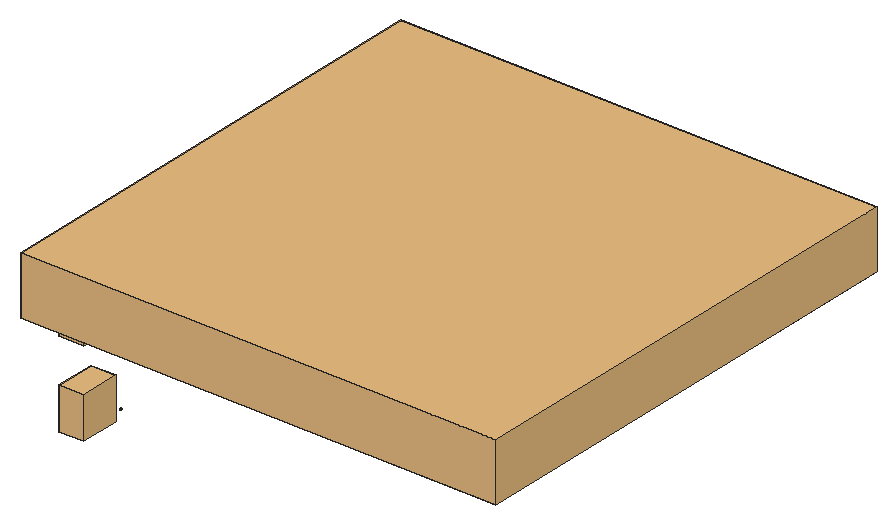
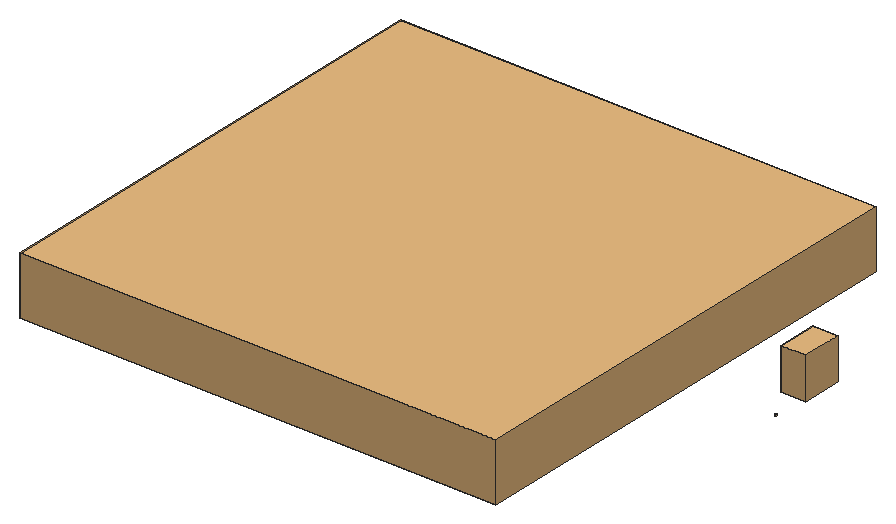
# SketchUp Ruby script. Lengths in inches.
U = 1.inch
M = Sketchup.active_model
def pt(a) = Geom::Point3d.new(a.map { |v| v * U })
def face(e, loops, mat)
  f = e.add_face(loops[0].map { |a| pt(a) })
  loops[1..].each { |l| e.add_face(l.map { |a| pt(a) }).erase! }
  f.material = f.back_material = mat if mat
  f
end
# faces: each face lists its corners as indices into pts; further lists are holes
def faces(e, pts, list, mat = nil) = list.each { |f| face(e, (f[0].is_a?(Array) ? f : [f]).map { |l| l.map { |i| pts[i] } }, mat) }
# xy, xz, yz: faces in a plane at the given z, y or x. An outline is a flat list of corners, or four numbers for a rectangle; further outlines are holes
def ring(l) = l.size == 4 ? [[l[0], l[1]], [l[2], l[1]], [l[2], l[3]], [l[0], l[3]]] : l.each_slice(2).to_a
def flat(e, list, mat, &to3) = list.each { |f| face(e, (f[0].is_a?(Array) ? f : [f]).map { |l| ring(l).map { |u, v| to3.(u, v) } }, mat) }
def xy(e, z, list, mat = nil) = flat(e, list, mat) { |x, y| [x, y, z] }
def xz(e, y, list, mat = nil) = flat(e, list, mat) { |x, z| [x, y, z] }
def yz(e, x, list, mat = nil) = flat(e, list, mat) { |y, z| [x, y, z] }
def lines(e, pts, list) = list.each { |a, b| e.add_line(pt(pts[a]), pt(pts[b])) }
# prism: a flat outline (further loops are holes) pulled along v
def prism(e, loops, v, mat = nil)
  f = face(e, loops, mat); d = Geom::Vector3d.new(v.map { |x| x * U })
  f.pushpull(f.normal.samedirection?(d) ? d.length : -d.length)
end
def box(e, o, s, mat = nil) = prism(e, [[o, [o[0] + s[0], o[1], o[2]], [o[0] + s[0], o[1] + s[1], o[2]], [o[0], o[1] + s[1], o[2]]]], [0, 0, s[2]], mat)
def at(x, y, z, deg = 0) = Geom::Transformation.translation(pt([x, y, z])) * Geom::Transformation.rotation(ORIGIN, Z_AXIS, deg.degrees)
def axes(o, x, y, z) = Geom::Transformation.new([*x, 0, *y, 0, *z, 0, *pt(o).to_a, 1])
def part(name) = M.definitions.add(name)
# library, detail: a bought-in or finely detailed component or shape, given as its bounding box
def library(name, o, s) = part(name).tap { |d| box(d.entities, o, s) }
def detail(e, o, s) = box(e.add_group.entities, o, s)
def put(e, d, t, mat = nil) = e.add_instance(d, t).tap { |i| i.material = mat if mat }
def group(e, t, mat = nil) = e.add_group.tap { |g| g.transformation = t; g.material = mat if mat }.entities
root = M.entities
M.materials.add("green").color = [174, 139, 102]
M.materials.add("vio").color = [206, 114, 100]
c1 = library("3DGeom~121_Defintion",[-425.32,-500,-417.04],[850.64,1000,834.08])
c2 = part("3DGeom~122_Defintion")
p = [[-352.95,-477.04,-406.33],[-422.05,-474.42,-360.32],[-383.91,-455.37,-417.04],[-352.95,-477.04,-406.33],[-383.91,-455.37,-417.04],[-365.48,-464.73,-416.07],
  [-383.91,-455.37,-417.04],[-422.05,-474.42,-360.32],[-418.46,-454.05,-394.04],[-383.91,-455.37,-417.04],[-418.46,-454.05,-394.04],[-403.3,-451.46,-408.98],
  [-356.54,-497.41,-372.61],[-422.05,-474.42,-360.32],[-352.95,-477.04,-406.33],[-356.54,-497.41,-372.61],[-352.95,-477.04,-406.33],[-349.67,-489,-390.42],
  [-422.05,-474.42,-360.32],[-425.32,-462.46,-376.23],[-418.46,-454.05,-394.04],[-391.09,-496.09,-349.6],[-356.54,-497.41,-372.61],[-371.7,-500,-357.67],
  [-391.09,-496.09,-349.6],[-422.05,-474.42,-360.32],[-356.54,-497.41,-372.61],[-422.05,-474.42,-360.32],[-391.09,-496.09,-349.6],[-409.52,-486.73,-350.57],
  [376.78,485.85,408.43],[420.34,458.37,345.52],[409.52,472.35,336.91],[376.78,485.85,408.43],[409.52,472.35,336.91],[395.77,486.26,339.03],
  [376.78,485.85,408.43],[395.77,486.26,339.03],[382.76,496.38,351.32],[376.78,485.85,408.43],[425.32,448.07,362.5625],[420.34,458.37,345.52],
  [376.78,485.85,408.43],[382.76,496.38,351.32],[373.99,500,370.48],[376.78,485.85,408.43],[423.13,444.22,383.47],[376.78,485.85,408.43],
  [373.99,500,370.48],[371.8,496.14,391.39],[376.78,485.85,408.43],[414.36,447.84,402.63],[423.13,444.22,383.47],[376.78,485.85,408.43],
  [401.35,457.96,414.92],[414.36,447.84,402.63],[376.78,485.85,408.43],[387.6,471.87,417.04],[401.35,457.96,414.92]]
faces(c2.entities,p,[[0,1,2],[3,4,5],[6,7,8],[9,10,11],[12,13,14],[15,16,17],[18,19,20],[21,22,23],
  [24,25,26],[27,28,29],[30,31,32],[33,34,35],[36,37,38],[39,40,41],[42,43,44],[45,46,40],
  [47,48,49],[50,51,52],[53,54,55],[56,57,58]],"green")
c3 = part("3DGeom~227_Defintion")
p = [[-46.82,-86.11,-495.11],[-183.22,-312.53,-297.48],[-255.21,-122.37,-414.37],[57.41,-270.66,-390.71],[148.25,12.96,-485.1875],[-138.51,121.52,-466.84],
  [-25.88,178.72,-461.11],[282.66,-156.27,-379.26],[277.73,148.29,-387.25],[48.875,256.85,-404.57],[-258.82,100.58,-420.23],[-193.08,296.58,-313.48],
  [-421.09,-86.11,-264.6],[-421.09,-86.11,-264.6],[-354.59,121.52,-333.75],[-255.21,-122.37,-414.37],[-183.22,-312.53,-297.48],[-374.76,-270.66,-124.54],
  [-255.21,-122.37,-414.37],[-421.09,-86.11,-264.6],[65.73,334.98,-312.37],[57.41,-270.66,-390.71],[-62.14,-418.95,-100.89],[-183.22,-312.53,-297.48],
  [57.41,-270.66,-390.71],[146.25,-382.69,-181.63],[146.25,-382.69,-181.63],[432.17,0,-266.17],[306.92,283.62,-227.56],[432.17,0,-266.17],
  [277.73,148.29,-387.25],[306.92,283.62,-227.56],[341.32,-283.625,-171.7],[146.25,-382.69,-181.63],[432.17,0,-266.17],[341.32,-283.625,-171.7],
  [282.66,-156.27,-379.26],[-354.59,121.52,-333.75],[-500,12.96,-85.92],[-354.59,121.52,-333.75],[-400.15,178.72,-230.6],[-400.15,178.72,-230.6],
  [-383.29,256.85,-138.4],[-193.08,296.58,-313.48],[-383.29,256.85,-138.4],[-308.54,334.98,-81.86],[-193.08,296.58,-313.48],[-195.91,392.18,-76.125],
  [-193.08,296.58,-313.48],[-75.6,413.11,-122.74],[-193.08,296.58,-313.48],[20.17,392.18,-209.21],[65.73,334.98,-312.37],[-193.08,296.58,-313.48],
  [-193.08,296.58,-313.48],[306.92,283.62,-227.56],[65.73,334.98,-312.37],[-183.22,-312.53,-297.48],[-228.01,-382.69,48.88],[-183.22,-312.53,-297.48],
  [-228.01,-382.69,48.88],[-374.76,-270.66,-124.54],[432.17,0,-266.17],[470.8,-148.29,-73.77],[341.32,-283.625,-171.7],[465.88,156.27,-81.77],
  [432.17,0,-266.17],[306.92,283.62,-227.56],[432.17,0,-266.17],[-465.88,-156.27,81.77],[-470.8,148.29,73.77],[-383.29,256.85,-138.4],
  [228.01,382.69,-48.88],[306.92,283.62,-227.56],[228.01,382.69,-48.88],[306.92,283.62,-227.56],[75.6,-413.11,122.74],[195.91,-392.18,76.125],
  [341.32,-283.625,-171.7],[341.32,-283.625,-171.7],[308.54,-334.98,81.86],[308.54,-334.98,81.86],[341.32,-283.625,-171.7],[-383.29,256.85,-138.4],
  [-341.32,283.625,171.7],[-383.29,256.85,-138.4],[-341.32,283.625,171.7],[-308.54,334.98,-81.86],[-228.01,-382.69,48.88],[-306.92,-283.62,227.56],
  [62.14,418.95,100.89],[-20.17,-392.18,209.21],[-228.01,-382.69,48.88],[-432.17,0,266.17],[-341.32,283.625,171.7],[-146.25,382.69,181.63],
  [500,-12.96,85.92],[374.76,270.66,124.54],[228.01,382.69,-48.88],[383.29,-256.85,138.4],[308.54,-334.98,81.86],[374.76,270.66,124.54],
  [-228.01,-382.69,48.88],[-65.73,-334.98,312.37],[-228.01,-382.69,48.88],[-65.73,-334.98,312.37],[-306.92,-283.62,227.56],[-282.66,156.27,379.26],
  [-282.66,156.27,379.26],[-341.32,283.625,171.7],[193.08,-296.58,313.48],[-277.73,-148.29,387.25],[-277.73,-148.29,387.25],[383.29,-256.85,138.4],
  [400.15,-178.72,230.6],[421.09,86.11,264.6],[183.22,312.53,297.48],[374.76,270.66,124.54],[183.22,312.53,297.48],[193.08,-296.58,313.48],
  [-341.32,283.625,171.7],[-282.66,156.27,379.26],[-57.41,270.66,390.71],[-341.32,283.625,171.7],[-57.41,270.66,390.71],[-146.25,382.69,181.63],
  [-57.41,270.66,390.71],[-65.73,-334.98,312.37],[-306.92,-283.62,227.56],[-65.73,-334.98,312.37],[-48.875,-256.85,404.57],[-306.92,-283.62,227.56],
  [-277.73,-148.29,387.25],[400.15,-178.72,230.6],[354.59,-121.52,333.75],[193.08,-296.58,313.48],[354.59,-121.52,333.75],[255.21,122.37,414.37],
  [354.59,-121.52,333.75],[421.09,86.11,264.6],[183.22,312.53,297.48],[255.21,122.37,414.37],[-432.17,0,266.17],[-148.25,-12.96,485.1875],
  [-432.17,0,266.17],[-57.41,270.66,390.71],[255.21,122.37,414.37],[183.22,312.53,297.48],[193.08,-296.58,313.48],[25.88,-178.72,461.11],
  [193.08,-296.58,313.48],[138.51,-121.52,466.84],[193.08,-296.58,313.48],[258.82,-100.58,420.23],[193.08,-296.58,313.48],[354.59,-121.52,333.75],
  [193.08,-296.58,313.48],[255.21,122.37,414.37],[354.59,-121.52,333.75],[46.82,86.11,495.11],[-57.41,270.66,390.71],[-57.41,270.66,390.71],
  [255.21,122.37,414.37],[255.21,122.37,414.37]]
faces(c3.entities,p,[[0,1,2],[0,3,1],[4,3,0],[5,0,2],[6,0,5],[6,4,0],[4,7,3],[8,7,4],
  [9,4,6],[9,8,4],[5,2,10],[5,10,11],[6,5,11],[9,6,11],[10,2,12],[10,13,14],
  [10,14,11],[15,16,17],[18,17,19],[20,8,9],[20,9,11],[21,22,23],[24,25,22],[7,26,3],
  [8,27,7],[28,29,30],[20,31,8],[7,32,33],[34,35,36],[37,19,38],[39,38,40],[14,41,11],
  [40,42,43],[44,45,46],[45,47,48],[47,49,50],[51,52,53],[49,51,54],[51,55,56],[57,22,58],
  [59,60,61],[62,63,64],[65,63,66],[67,65,68],[19,17,69],[19,69,38],[40,38,70],[40,70,71],
  [72,65,73],[51,74,75],[49,74,51],[25,76,22],[25,77,76],[78,77,25],[79,80,77],[63,81,82],
  [83,70,84],[85,86,87],[17,88,89],[17,89,69],[49,90,74],[47,90,49],[22,91,92],[22,76,91],
  [38,69,93],[38,93,70],[45,94,95],[45,95,47],[65,96,63],[97,96,65],[98,97,65],[47,95,90],
  [63,99,100],[96,99,63],[90,101,74],[102,91,103],[104,105,106],[70,93,107],[70,108,109],[76,77,110],
  [77,80,110],[69,89,111],[69,112,93],[80,113,110],[96,114,99],[115,114,96],[97,115,96],[90,116,117],
  [95,116,90],[91,76,110],[118,115,97],[99,114,119],[120,121,122],[123,124,125],[95,126,116],[127,91,110],
  [128,129,130],[131,130,132],[133,134,135],[115,136,114],[137,138,139],[140,141,115],[142,132,143],[144,143,121],
  [145,146,147],[130,129,148],[149,130,150],[151,149,152],[153,151,154],[155,153,156],[157,153,158],[121,143,159],
  [121,159,160],[132,130,149],[132,149,143],[161,159,162],[159,153,163],[159,151,153],[143,149,151],[143,151,159]],"vio")
c4 = library("plants1",[-17.48,-17.55,0],[53.57,32.72,56.26])
c5 = library("Marble Pot Grass",[0.11,0.16,0],[7.58,7.55,8.56])
c6 = library("living false ceiling",[271.93,40.8,71.63],[192,192,23.47])
g1 = group(root,at(15.3125,38.42,26.21))
put(g1,c1,axes([4.85,0.57,15.95],[0,0.00036,0],[0,0,-0.00036],[-0.00036,0,0]),"green")
put(g1,c2,axes([4.85,0.57,15.95],[0,0.00036,0],[0,0,-0.00036],[-0.00036,0,0]),"green")
g2 = group(root,at(15.3125,38.42,26.21))
put(g2,c3,axes([5.01,0.41,16.15],[0,0.00038,0],[0,0,-0.00038],[-0.00038,0,0]),"vio")
put(root,c4,axes([20.73,18.17,44],[0,0.3,0],[-0.3,0,0],[0,0,0.3]))
put(root,c4,axes([21.45,23.76,78.5],[0,-0.3,0],[0.3,0,0],[0,0,0.3]))
put(root,c5,at(26,37.34,79.5,90))
put(root,c6,at(238.8,-265.93,12.9,90))
